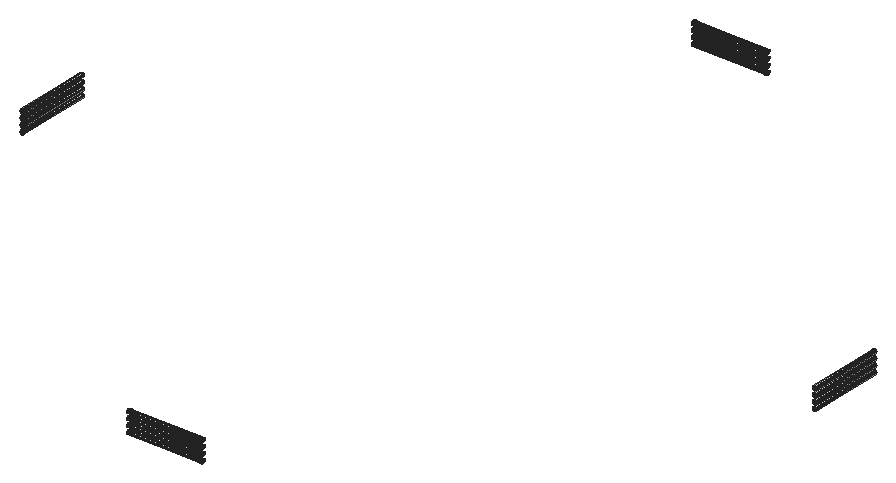
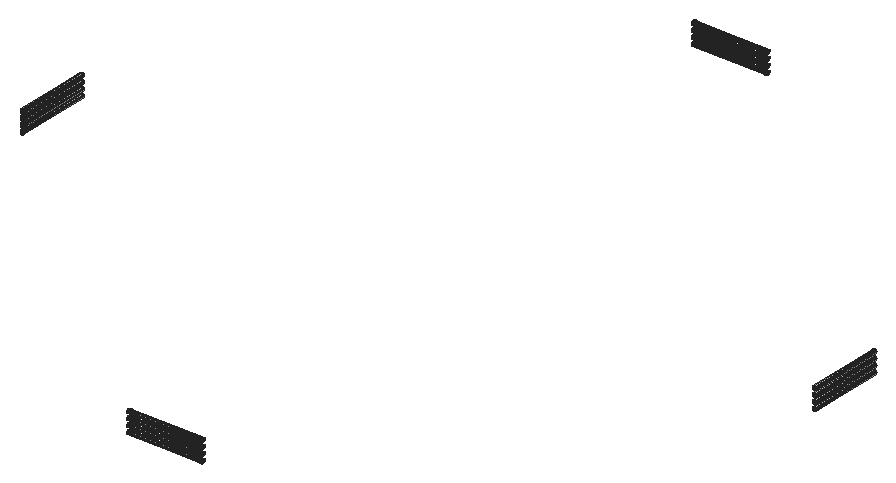
# SketchUp Ruby script. Lengths in inches.
U = 1.inch
M = Sketchup.active_model
def pt(a) = Geom::Point3d.new(a.map { |v| v * U })
def face(e, loops, mat)
  f = e.add_face(loops[0].map { |a| pt(a) })
  loops[1..].each { |l| e.add_face(l.map { |a| pt(a) }).erase! }
  f.material = f.back_material = mat if mat
  f
end
# faces: each face lists its corners as indices into pts; further lists are holes
def faces(e, pts, list, mat = nil) = list.each { |f| face(e, (f[0].is_a?(Array) ? f : [f]).map { |l| l.map { |i| pts[i] } }, mat) }
# xy, xz, yz: faces in a plane at the given z, y or x. An outline is a flat list of corners, or four numbers for a rectangle; further outlines are holes
def ring(l) = l.size == 4 ? [[l[0], l[1]], [l[2], l[1]], [l[2], l[3]], [l[0], l[3]]] : l.each_slice(2).to_a
def flat(e, list, mat, &to3) = list.each { |f| face(e, (f[0].is_a?(Array) ? f : [f]).map { |l| ring(l).map { |u, v| to3.(u, v) } }, mat) }
def xy(e, z, list, mat = nil) = flat(e, list, mat) { |x, y| [x, y, z] }
def xz(e, y, list, mat = nil) = flat(e, list, mat) { |x, z| [x, y, z] }
def yz(e, x, list, mat = nil) = flat(e, list, mat) { |y, z| [x, y, z] }
def lines(e, pts, list) = list.each { |a, b| e.add_line(pt(pts[a]), pt(pts[b])) }
# prism: a flat outline (further loops are holes) pulled along v
def prism(e, loops, v, mat = nil)
  f = face(e, loops, mat); d = Geom::Vector3d.new(v.map { |x| x * U })
  f.pushpull(f.normal.samedirection?(d) ? d.length : -d.length)
end
def box(e, o, s, mat = nil) = prism(e, [[o, [o[0] + s[0], o[1], o[2]], [o[0] + s[0], o[1] + s[1], o[2]], [o[0], o[1] + s[1], o[2]]]], [0, 0, s[2]], mat)
def at(x, y, z, deg = 0) = Geom::Transformation.translation(pt([x, y, z])) * Geom::Transformation.rotation(ORIGIN, Z_AXIS, deg.degrees)
def axes(o, x, y, z) = Geom::Transformation.new([*x, 0, *y, 0, *z, 0, *pt(o).to_a, 1])
def part(name) = M.definitions.add(name)
# library, detail: a bought-in or finely detailed component or shape, given as its bounding box
def library(name, o, s) = part(name).tap { |d| box(d.entities, o, s) }
def detail(e, o, s) = box(e.add_group.entities, o, s)
def put(e, d, t, mat = nil) = e.add_instance(d, t).tap { |i| i.material = mat if mat }
def group(e, t, mat = nil) = e.add_group.tap { |g| g.transformation = t; g.material = mat if mat }.entities
root = M.entities
p = [[922.01,48.34,1269.02],[922.01,47.38,1269.14],[778.64,47.38,1269.14],[778.64,48.34,1269.02],[922.01,49.29,1269.14],[778.64,49.29,1269.14],
  [83.53,662.8,1269.02],[82.57,662.8,1269.14],[82.57,806.17,1269.14],[83.53,806.17,1269.02],[84.48,662.8,1269.14],[84.48,806.17,1269.14],
  [1535.52,886.83,1269.14],[1536.47,886.83,1269.02],[1536.47,743.45,1269.02],[1535.52,743.45,1269.14],[1537.43,886.83,1269.14],[1537.43,743.45,1269.14],
  [697.99,1500.33,1269.14],[697.99,1501.28,1269.02],[841.36,1501.28,1269.02],[841.36,1500.33,1269.14],[697.99,1502.24,1269.14],[841.36,1502.24,1269.14],
  [922.01,46.5,1269.51],[778.64,46.5,1269.51],[922.01,50.18,1269.51],[778.64,50.18,1269.51],[81.68,662.8,1269.51],[81.68,806.17,1269.51],
  [85.37,662.8,1269.51],[85.37,806.17,1269.51],[1534.63,886.83,1269.51],[1534.63,743.45,1269.51],[1538.32,886.83,1269.51],[1538.32,743.45,1269.51],
  [697.99,1499.44,1269.51],[841.36,1499.44,1269.51],[697.99,1503.13,1269.51],[841.36,1503.13,1269.51],[922.01,45.73,1270.1],[778.64,45.73,1270.1],
  [922.01,50.95,1270.1],[778.64,50.95,1270.1],[80.92,662.8,1270.1],[80.92,806.17,1270.1],[86.13,662.8,1270.1],[86.13,806.17,1270.1],
  [1533.87,886.83,1270.1],[1533.87,743.45,1270.1],[1539.08,886.83,1270.1],[1539.08,743.45,1270.1],[697.99,1498.68,1270.1],[841.36,1498.68,1270.1],
  [697.99,1503.89,1270.1],[841.36,1503.89,1270.1],[922.01,45.15,1270.86],[778.64,45.15,1270.86],[922.01,51.53,1270.86],[778.64,51.53,1270.86],
  [80.33,662.8,1270.86],[80.33,806.17,1270.86],[86.72,662.8,1270.86],[86.72,806.17,1270.86],[1533.28,886.83,1270.86],[1533.28,743.45,1270.86],
  [1539.67,886.83,1270.86],[1539.67,743.45,1270.86],[697.99,1498.09,1270.86],[841.36,1498.09,1270.86],[697.99,1504.48,1270.86],[841.36,1504.48,1270.86],
  [922.01,44.78,1271.75],[778.64,44.78,1271.75],[922.01,51.9,1271.75],[778.64,51.9,1271.75],[79.97,662.8,1271.75],[79.97,806.17,1271.75],
  [87.09,662.8,1271.75],[87.09,806.17,1271.75],[1532.91,886.83,1271.75],[1532.91,743.45,1271.75],[1540.03,886.83,1271.75],[1540.03,743.45,1271.75],
  [697.99,1497.72,1271.75],[841.36,1497.72,1271.75],[697.99,1504.85,1271.75],[841.36,1504.85,1271.75],[922.01,44.65,1272.7],[778.64,44.65,1272.7],
  [922.01,52.03,1272.7],[778.64,52.03,1272.7],[79.84,662.8,1272.7],[79.84,806.17,1272.7],[87.21,662.8,1272.7],[87.21,806.17,1272.7],
  [1532.79,886.83,1272.7],[1532.79,743.45,1272.7],[1540.16,886.83,1272.7],[1540.16,743.45,1272.7],[697.99,1497.6,1272.7],[841.36,1497.6,1272.7],
  [697.99,1504.97,1272.7],[841.36,1504.97,1272.7],[922.01,44.78,1273.66],[778.64,44.78,1273.66],[922.01,51.9,1273.66],[778.64,51.9,1273.66],
  [79.97,662.8,1273.66],[79.97,806.17,1273.66],[87.09,662.8,1273.66],[87.09,806.17,1273.66],[1532.91,886.83,1273.66],[1532.91,743.45,1273.66],
  [1540.03,886.83,1273.66],[1540.03,743.45,1273.66],[697.99,1497.72,1273.66],[841.36,1497.72,1273.66],[697.99,1504.85,1273.66],[841.36,1504.85,1273.66],
  [922.01,45.15,1274.55],[778.64,45.15,1274.55],[922.01,51.53,1274.55],[778.64,51.53,1274.55],[80.33,662.8,1274.55],[80.33,806.17,1274.55],
  [86.72,662.8,1274.55],[86.72,806.17,1274.55],[1533.28,886.83,1274.55],[1533.28,743.45,1274.55],[1539.67,886.83,1274.55],[1539.67,743.45,1274.55],
  [697.99,1498.09,1274.55],[841.36,1498.09,1274.55],[697.99,1504.48,1274.55],[841.36,1504.48,1274.55],[922.01,45.73,1275.3125],[778.64,45.73,1275.3125],
  [922.01,50.95,1275.3125],[778.64,50.95,1275.3125],[80.92,662.8,1275.3125],[80.92,806.17,1275.3125],[86.13,662.8,1275.3125],[86.13,806.17,1275.3125],
  [1533.87,886.83,1275.3125],[1533.87,743.45,1275.3125],[1539.08,886.83,1275.3125],[1539.08,743.45,1275.3125],[697.99,1498.68,1275.3125],[841.36,1498.68,1275.3125],
  [697.99,1503.89,1275.3125],[841.36,1503.89,1275.3125],[922.01,46.5,1275.9],[778.64,46.5,1275.9],[922.01,50.18,1275.9],[778.64,50.18,1275.9],
  [81.68,662.8,1275.9],[81.68,806.17,1275.9],[85.37,662.8,1275.9],[85.37,806.17,1275.9],[1534.63,886.83,1275.9],[1534.63,743.45,1275.9],
  [1538.32,886.83,1275.9],[1538.32,743.45,1275.9],[697.99,1499.44,1275.9],[841.36,1499.44,1275.9],[697.99,1503.13,1275.9],[841.36,1503.13,1275.9],
  [922.01,47.38,1276.27],[778.64,47.38,1276.27],[922.01,49.29,1276.27],[778.64,49.29,1276.27],[82.57,662.8,1276.27],[82.57,806.17,1276.27],
  [84.48,662.8,1276.27],[84.48,806.17,1276.27],[1535.52,886.83,1276.27],[1535.52,743.45,1276.27],[1537.43,886.83,1276.27],[1537.43,743.45,1276.27],
  [697.99,1500.33,1276.27],[841.36,1500.33,1276.27],[697.99,1502.24,1276.27],[841.36,1502.24,1276.27],[922.01,48.34,1276.39],[778.64,48.34,1276.39],
  [83.53,662.8,1276.39],[83.53,806.17,1276.39],[1536.47,886.83,1276.39],[1536.47,743.45,1276.39],[697.99,1501.28,1276.39],[841.36,1501.28,1276.39],
  [922.01,48.34,1281.02],[922.01,47.38,1281.14],[778.64,47.38,1281.14],[778.64,48.34,1281.02],[922.01,49.29,1281.14],[778.64,49.29,1281.14],
  [83.53,662.8,1281.02],[82.57,662.8,1281.14],[82.57,806.17,1281.14],[83.53,806.17,1281.02],[84.48,662.8,1281.14],[84.48,806.17,1281.14],
  [1535.52,886.83,1281.14],[1536.47,886.83,1281.02],[1536.47,743.45,1281.02],[1535.52,743.45,1281.14],[1537.43,886.83,1281.14],[1537.43,743.45,1281.14],
  [697.99,1500.33,1281.14],[697.99,1501.28,1281.02],[841.36,1501.28,1281.02],[841.36,1500.33,1281.14],[697.99,1502.24,1281.14],[841.36,1502.24,1281.14],
  [922.01,46.5,1281.51],[778.64,46.5,1281.51],[922.01,50.18,1281.51],[778.64,50.18,1281.51],[81.68,662.8,1281.51],[81.68,806.17,1281.51],
  [85.37,662.8,1281.51],[85.37,806.17,1281.51],[1534.63,886.83,1281.51],[1534.63,743.45,1281.51],[1538.32,886.83,1281.51],[1538.32,743.45,1281.51],
  [697.99,1499.44,1281.51],[841.36,1499.44,1281.51],[697.99,1503.13,1281.51],[841.36,1503.13,1281.51],[922.01,45.73,1282.1],[778.64,45.73,1282.1],
  [922.01,50.95,1282.1],[778.64,50.95,1282.1],[80.92,662.8,1282.1],[80.92,806.17,1282.1],[86.13,662.8,1282.1],[86.13,806.17,1282.1],
  [1533.87,886.83,1282.1],[1533.87,743.45,1282.1],[1539.08,886.83,1282.1],[1539.08,743.45,1282.1],[697.99,1498.68,1282.1],[841.36,1498.68,1282.1],
  [697.99,1503.89,1282.1],[841.36,1503.89,1282.1],[922.01,45.15,1282.86],[778.64,45.15,1282.86],[922.01,51.53,1282.86],[778.64,51.53,1282.86],
  [80.33,662.8,1282.86],[80.33,806.17,1282.86],[86.72,662.8,1282.86],[86.72,806.17,1282.86],[1533.28,886.83,1282.86],[1533.28,743.45,1282.86],
  [1539.67,886.83,1282.86],[1539.67,743.45,1282.86],[697.99,1498.09,1282.86],[841.36,1498.09,1282.86],[697.99,1504.48,1282.86],[841.36,1504.48,1282.86],
  [922.01,44.78,1283.75],[778.64,44.78,1283.75],[922.01,51.9,1283.75],[778.64,51.9,1283.75],[79.97,662.8,1283.75],[79.97,806.17,1283.75],
  [87.09,662.8,1283.75],[87.09,806.17,1283.75],[1532.91,886.83,1283.75],[1532.91,743.45,1283.75],[1540.03,886.83,1283.75],[1540.03,743.45,1283.75],
  [697.99,1497.72,1283.75],[841.36,1497.72,1283.75],[697.99,1504.85,1283.75],[841.36,1504.85,1283.75],[922.01,44.65,1284.7],[778.64,44.65,1284.7],
  [922.01,52.03,1284.7],[778.64,52.03,1284.7],[79.84,662.8,1284.7],[79.84,806.17,1284.7],[87.21,662.8,1284.7],[87.21,806.17,1284.7],
  [1532.79,886.83,1284.7],[1532.79,743.45,1284.7],[1540.16,886.83,1284.7],[1540.16,743.45,1284.7],[697.99,1497.6,1284.7],[841.36,1497.6,1284.7],
  [697.99,1504.97,1284.7],[841.36,1504.97,1284.7],[922.01,44.78,1285.66],[778.64,44.78,1285.66],[922.01,51.9,1285.66],[778.64,51.9,1285.66],
  [79.97,662.8,1285.66],[79.97,806.17,1285.66],[87.09,662.8,1285.66],[87.09,806.17,1285.66],[1532.91,886.83,1285.66],[1532.91,743.45,1285.66],
  [1540.03,886.83,1285.66],[1540.03,743.45,1285.66],[697.99,1497.72,1285.66],[841.36,1497.72,1285.66],[697.99,1504.85,1285.66],[841.36,1504.85,1285.66],
  [922.01,45.15,1286.55],[778.64,45.15,1286.55],[922.01,51.53,1286.55],[778.64,51.53,1286.55],[80.33,662.8,1286.55],[80.33,806.17,1286.55],
  [86.72,662.8,1286.55],[86.72,806.17,1286.55],[1533.28,886.83,1286.55],[1533.28,743.45,1286.55],[1539.67,886.83,1286.55],[1539.67,743.45,1286.55],
  [697.99,1498.09,1286.55],[841.36,1498.09,1286.55],[697.99,1504.48,1286.55],[841.36,1504.48,1286.55],[922.01,45.73,1287.3125],[778.64,45.73,1287.3125],
  [922.01,50.95,1287.3125],[778.64,50.95,1287.3125],[80.92,662.8,1287.3125],[80.92,806.17,1287.3125],[86.13,662.8,1287.3125],[86.13,806.17,1287.3125],
  [1533.87,886.83,1287.3125],[1533.87,743.45,1287.3125],[1539.08,886.83,1287.3125],[1539.08,743.45,1287.3125],[697.99,1498.68,1287.3125],[841.36,1498.68,1287.3125],
  [697.99,1503.89,1287.3125],[841.36,1503.89,1287.3125],[922.01,46.5,1287.9],[778.64,46.5,1287.9],[922.01,50.18,1287.9],[778.64,50.18,1287.9],
  [81.68,662.8,1287.9],[81.68,806.17,1287.9],[85.37,662.8,1287.9],[85.37,806.17,1287.9],[1534.63,886.83,1287.9],[1534.63,743.45,1287.9],
  [1538.32,886.83,1287.9],[1538.32,743.45,1287.9],[697.99,1499.44,1287.9],[841.36,1499.44,1287.9],[697.99,1503.13,1287.9],[841.36,1503.13,1287.9],
  [922.01,47.38,1288.27],[778.64,47.38,1288.27],[922.01,49.29,1288.27],[778.64,49.29,1288.27],[82.57,662.8,1288.27],[82.57,806.17,1288.27],
  [84.48,662.8,1288.27],[84.48,806.17,1288.27],[1535.52,886.83,1288.27],[1535.52,743.45,1288.27],[1537.43,886.83,1288.27],[1537.43,743.45,1288.27],
  [697.99,1500.33,1288.27],[841.36,1500.33,1288.27],[697.99,1502.24,1288.27],[841.36,1502.24,1288.27],[922.01,48.34,1288.39],[778.64,48.34,1288.39],
  [83.53,662.8,1288.39],[83.53,806.17,1288.39],[1536.47,886.83,1288.39],[1536.47,743.45,1288.39],[697.99,1501.28,1288.39],[841.36,1501.28,1288.39],
  [922.01,48.34,1293.02],[922.01,47.38,1293.14],[778.64,47.38,1293.14],[778.64,48.34,1293.02],[922.01,49.29,1293.14],[778.64,49.29,1293.14],
  [83.53,662.8,1293.02],[82.57,662.8,1293.14],[82.57,806.17,1293.14],[83.53,806.17,1293.02],[84.48,662.8,1293.14],[84.48,806.17,1293.14],
  [1535.52,886.83,1293.14],[1536.47,886.83,1293.02],[1536.47,743.45,1293.02],[1535.52,743.45,1293.14],[1537.43,886.83,1293.14],[1537.43,743.45,1293.14],
  [697.99,1500.33,1293.14],[697.99,1501.28,1293.02],[841.36,1501.28,1293.02],[841.36,1500.33,1293.14],[697.99,1502.24,1293.14],[841.36,1502.24,1293.14],
  [922.01,46.5,1293.51],[778.64,46.5,1293.51],[922.01,50.18,1293.51],[778.64,50.18,1293.51],[81.68,662.8,1293.51],[81.68,806.17,1293.51],
  [85.37,662.8,1293.51],[85.37,806.17,1293.51],[1534.63,886.83,1293.51],[1534.63,743.45,1293.51],[1538.32,886.83,1293.51],[1538.32,743.45,1293.51],
  [697.99,1499.44,1293.51],[841.36,1499.44,1293.51],[697.99,1503.13,1293.51],[841.36,1503.13,1293.51],[922.01,45.73,1294.1],[778.64,45.73,1294.1],
  [922.01,50.95,1294.1],[778.64,50.95,1294.1],[80.92,662.8,1294.1],[80.92,806.17,1294.1],[86.13,662.8,1294.1],[86.13,806.17,1294.1],
  [1533.87,886.83,1294.1],[1533.87,743.45,1294.1],[1539.08,886.83,1294.1],[1539.08,743.45,1294.1],[697.99,1498.68,1294.1],[841.36,1498.68,1294.1],
  [697.99,1503.89,1294.1],[841.36,1503.89,1294.1],[922.01,45.15,1294.86],[778.64,45.15,1294.86],[922.01,51.53,1294.86],[778.64,51.53,1294.86],
  [80.33,662.8,1294.86],[80.33,806.17,1294.86],[86.72,662.8,1294.86],[86.72,806.17,1294.86],[1533.28,886.83,1294.86],[1533.28,743.45,1294.86],
  [1539.67,886.83,1294.86],[1539.67,743.45,1294.86],[697.99,1498.09,1294.86],[841.36,1498.09,1294.86],[697.99,1504.48,1294.86],[841.36,1504.48,1294.86],
  [922.01,44.78,1295.75],[778.64,44.78,1295.75],[922.01,51.9,1295.75],[778.64,51.9,1295.75],[79.97,662.8,1295.75],[79.97,806.17,1295.75],
  [87.09,662.8,1295.75],[87.09,806.17,1295.75],[1532.91,886.83,1295.75],[1532.91,743.45,1295.75],[1540.03,886.83,1295.75],[1540.03,743.45,1295.75],
  [697.99,1497.72,1295.75],[841.36,1497.72,1295.75],[697.99,1504.85,1295.75],[841.36,1504.85,1295.75],[922.01,44.65,1296.7],[778.64,44.65,1296.7],
  [922.01,52.03,1296.7],[778.64,52.03,1296.7],[79.84,662.8,1296.7],[79.84,806.17,1296.7],[87.21,662.8,1296.7],[87.21,806.17,1296.7],
  [1532.79,886.83,1296.7],[1532.79,743.45,1296.7],[1540.16,886.83,1296.7],[1540.16,743.45,1296.7],[697.99,1497.6,1296.7],[841.36,1497.6,1296.7],
  [697.99,1504.97,1296.7],[841.36,1504.97,1296.7],[922.01,44.78,1297.66],[778.64,44.78,1297.66],[922.01,51.9,1297.66],[778.64,51.9,1297.66],
  [79.97,662.8,1297.66],[79.97,806.17,1297.66],[87.09,662.8,1297.66],[87.09,806.17,1297.66],[1532.91,886.83,1297.66],[1532.91,743.45,1297.66],
  [1540.03,886.83,1297.66],[1540.03,743.45,1297.66],[697.99,1497.72,1297.66],[841.36,1497.72,1297.66],[697.99,1504.85,1297.66],[841.36,1504.85,1297.66],
  [922.01,45.15,1298.55],[778.64,45.15,1298.55],[922.01,51.53,1298.55],[778.64,51.53,1298.55],[80.33,662.8,1298.55],[80.33,806.17,1298.55],
  [86.72,662.8,1298.55],[86.72,806.17,1298.55],[1533.28,886.83,1298.55],[1533.28,743.45,1298.55],[1539.67,886.83,1298.55],[1539.67,743.45,1298.55],
  [697.99,1498.09,1298.55],[841.36,1498.09,1298.55],[697.99,1504.48,1298.55],[841.36,1504.48,1298.55],[922.01,45.73,1299.3125],[778.64,45.73,1299.3125],
  [922.01,50.95,1299.3125],[778.64,50.95,1299.3125],[80.92,662.8,1299.3125],[80.92,806.17,1299.3125],[86.13,662.8,1299.3125],[86.13,806.17,1299.3125],
  [1533.87,886.83,1299.3125],[1533.87,743.45,1299.3125],[1539.08,886.83,1299.3125],[1539.08,743.45,1299.3125],[697.99,1498.68,1299.3125],[841.36,1498.68,1299.3125],
  [697.99,1503.89,1299.3125],[841.36,1503.89,1299.3125],[922.01,46.5,1299.9],[778.64,46.5,1299.9],[922.01,50.18,1299.9],[778.64,50.18,1299.9],
  [81.68,662.8,1299.9],[81.68,806.17,1299.9],[85.37,662.8,1299.9],[85.37,806.17,1299.9],[1534.63,886.83,1299.9],[1534.63,743.45,1299.9],
  [1538.32,886.83,1299.9],[1538.32,743.45,1299.9],[697.99,1499.44,1299.9],[841.36,1499.44,1299.9],[697.99,1503.13,1299.9],[841.36,1503.13,1299.9],
  [922.01,47.38,1300.27],[778.64,47.38,1300.27],[922.01,49.29,1300.27],[778.64,49.29,1300.27],[82.57,662.8,1300.27],[82.57,806.17,1300.27],
  [84.48,662.8,1300.27],[84.48,806.17,1300.27],[1535.52,886.83,1300.27],[1535.52,743.45,1300.27],[1537.43,886.83,1300.27],[1537.43,743.45,1300.27],
  [697.99,1500.33,1300.27],[841.36,1500.33,1300.27],[697.99,1502.24,1300.27],[841.36,1502.24,1300.27],[922.01,48.34,1300.39],[778.64,48.34,1300.39],
  [83.53,662.8,1300.39],[83.53,806.17,1300.39],[1536.47,886.83,1300.39],[1536.47,743.45,1300.39],[697.99,1501.28,1300.39],[841.36,1501.28,1300.39],
  [922.01,48.34,1305.02],[922.01,47.38,1305.14],[778.64,47.38,1305.14],[778.64,48.34,1305.02],[922.01,49.29,1305.14],[778.64,49.29,1305.14],
  [83.53,662.8,1305.02],[82.57,662.8,1305.14],[82.57,806.17,1305.14],[83.53,806.17,1305.02],[84.48,662.8,1305.14],[84.48,806.17,1305.14],
  [1535.52,886.83,1305.14],[1536.47,886.83,1305.02],[1536.47,743.45,1305.02],[1535.52,743.45,1305.14],[1537.43,886.83,1305.14],[1537.43,743.45,1305.14],
  [697.99,1500.33,1305.14],[697.99,1501.28,1305.02],[841.36,1501.28,1305.02],[841.36,1500.33,1305.14],[697.99,1502.24,1305.14],[841.36,1502.24,1305.14],
  [922.01,46.5,1305.51],[778.64,46.5,1305.51],[922.01,50.18,1305.51],[778.64,50.18,1305.51],[81.68,662.8,1305.51],[81.68,806.17,1305.51],
  [85.37,662.8,1305.51],[85.37,806.17,1305.51],[1534.63,886.83,1305.51],[1534.63,743.45,1305.51],[1538.32,886.83,1305.51],[1538.32,743.45,1305.51],
  [697.99,1499.44,1305.51],[841.36,1499.44,1305.51],[697.99,1503.13,1305.51],[841.36,1503.13,1305.51],[922.01,45.73,1306.1],[778.64,45.73,1306.1],
  [922.01,50.95,1306.1],[778.64,50.95,1306.1],[80.92,662.8,1306.1],[80.92,806.17,1306.1],[86.13,662.8,1306.1],[86.13,806.17,1306.1],
  [1533.87,886.83,1306.1],[1533.87,743.45,1306.1],[1539.08,886.83,1306.1],[1539.08,743.45,1306.1],[697.99,1498.68,1306.1],[841.36,1498.68,1306.1],
  [697.99,1503.89,1306.1],[841.36,1503.89,1306.1],[922.01,45.15,1306.86],[778.64,45.15,1306.86],[922.01,51.53,1306.86],[778.64,51.53,1306.86],
  [80.33,662.8,1306.86],[80.33,806.17,1306.86],[86.72,662.8,1306.86],[86.72,806.17,1306.86],[1533.28,886.83,1306.86],[1533.28,743.45,1306.86],
  [1539.67,886.83,1306.86],[1539.67,743.45,1306.86],[697.99,1498.09,1306.86],[841.36,1498.09,1306.86],[697.99,1504.48,1306.86],[841.36,1504.48,1306.86],
  [922.01,44.78,1307.75],[778.64,44.78,1307.75],[922.01,51.9,1307.75],[778.64,51.9,1307.75],[79.97,662.8,1307.75],[79.97,806.17,1307.75],
  [87.09,662.8,1307.75],[87.09,806.17,1307.75],[1532.91,886.83,1307.75],[1532.91,743.45,1307.75],[1540.03,886.83,1307.75],[1540.03,743.45,1307.75],
  [697.99,1497.72,1307.75],[841.36,1497.72,1307.75],[697.99,1504.85,1307.75],[841.36,1504.85,1307.75],[922.01,44.65,1308.7],[778.64,44.65,1308.7],
  [922.01,52.03,1308.7],[778.64,52.03,1308.7],[79.84,662.8,1308.7],[79.84,806.17,1308.7],[87.21,662.8,1308.7],[87.21,806.17,1308.7],
  [1532.79,886.83,1308.7],[1532.79,743.45,1308.7],[1540.16,886.83,1308.7],[1540.16,743.45,1308.7],[697.99,1497.6,1308.7],[841.36,1497.6,1308.7],
  [697.99,1504.97,1308.7],[841.36,1504.97,1308.7],[922.01,44.78,1309.66],[778.64,44.78,1309.66],[922.01,51.9,1309.66],[778.64,51.9,1309.66],
  [79.97,662.8,1309.66],[79.97,806.17,1309.66],[87.09,662.8,1309.66],[87.09,806.17,1309.66],[1532.91,886.83,1309.66],[1532.91,743.45,1309.66],
  [1540.03,886.83,1309.66],[1540.03,743.45,1309.66],[697.99,1497.72,1309.66],[841.36,1497.72,1309.66],[697.99,1504.85,1309.66],[841.36,1504.85,1309.66],
  [922.01,45.15,1310.55],[778.64,45.15,1310.55],[922.01,51.53,1310.55],[778.64,51.53,1310.55],[80.33,662.8,1310.55],[80.33,806.17,1310.55],
  [86.72,662.8,1310.55],[86.72,806.17,1310.55],[1533.28,886.83,1310.55],[1533.28,743.45,1310.55],[1539.67,886.83,1310.55],[1539.67,743.45,1310.55],
  [697.99,1498.09,1310.55],[841.36,1498.09,1310.55],[697.99,1504.48,1310.55],[841.36,1504.48,1310.55],[922.01,45.73,1311.3125],[778.64,45.73,1311.3125],
  [922.01,50.95,1311.3125],[778.64,50.95,1311.3125],[80.92,662.8,1311.3125],[80.92,806.17,1311.3125],[86.13,662.8,1311.3125],[86.13,806.17,1311.3125],
  [1533.87,886.83,1311.3125],[1533.87,743.45,1311.3125],[1539.08,886.83,1311.3125],[1539.08,743.45,1311.3125],[697.99,1498.68,1311.3125],[841.36,1498.68,1311.3125],
  [697.99,1503.89,1311.3125],[841.36,1503.89,1311.3125],[922.01,46.5,1311.9],[778.64,46.5,1311.9],[922.01,50.18,1311.9],[778.64,50.18,1311.9],
  [81.68,662.8,1311.9],[81.68,806.17,1311.9],[85.37,662.8,1311.9],[85.37,806.17,1311.9],[1534.63,886.83,1311.9],[1534.63,743.45,1311.9],
  [1538.32,886.83,1311.9],[1538.32,743.45,1311.9],[697.99,1499.44,1311.9],[841.36,1499.44,1311.9],[697.99,1503.13,1311.9],[841.36,1503.13,1311.9],
  [922.01,47.38,1312.27],[778.64,47.38,1312.27],[922.01,49.29,1312.27],[778.64,49.29,1312.27],[82.57,662.8,1312.27],[82.57,806.17,1312.27],
  [84.48,662.8,1312.27],[84.48,806.17,1312.27],[1535.52,886.83,1312.27],[1535.52,743.45,1312.27],[1537.43,886.83,1312.27],[1537.43,743.45,1312.27],
  [697.99,1500.33,1312.27],[841.36,1500.33,1312.27],[697.99,1502.24,1312.27],[841.36,1502.24,1312.27],[922.01,48.34,1312.39],[778.64,48.34,1312.39],
  [83.53,662.8,1312.39],[83.53,806.17,1312.39],[1536.47,886.83,1312.39],[1536.47,743.45,1312.39],[697.99,1501.28,1312.39],[841.36,1501.28,1312.39]]
faces(root,p,[[0,1,2,3],[4,0,3,5],[6,7,8,9],[10,6,9,11],[12,13,14,15],[13,16,17,14],[18,19,20,21],[19,22,23,20],
  [1,24,25,2],[26,4,5,27],[7,28,29,8],[30,10,11,31],[32,12,15,33],[16,34,35,17],[36,18,21,37],[22,38,39,23],
  [24,40,41,25],[42,26,27,43],[28,44,45,29],[46,30,31,47],[48,32,33,49],[34,50,51,35],[52,36,37,53],[38,54,55,39],
  [40,56,57,41],[58,42,43,59],[44,60,61,45],[62,46,47,63],[64,48,49,65],[50,66,67,51],[68,52,53,69],[54,70,71,55],
  [56,72,73,57],[74,58,59,75],[60,76,77,61],[78,62,63,79],[80,64,65,81],[66,82,83,67],[84,68,69,85],[70,86,87,71],
  [72,88,89,73],[90,74,75,91],[76,92,93,77],[94,78,79,95],[96,80,81,97],[82,98,99,83],[100,84,85,101],[86,102,103,87],
  [88,104,105,89],[106,90,91,107],[92,108,109,93],[110,94,95,111],[112,96,97,113],[98,114,115,99],[116,100,101,117],[102,118,119,103],
  [104,120,121,105],[122,106,107,123],[108,124,125,109],[126,110,111,127],[128,112,113,129],[114,130,131,115],[132,116,117,133],[118,134,135,119],
  [120,136,137,121],[138,122,123,139],[124,140,141,125],[142,126,127,143],[144,128,129,145],[130,146,147,131],[148,132,133,149],[134,150,151,135],
  [136,152,153,137],[154,138,139,155],[140,156,157,141],[158,142,143,159],[160,144,145,161],[146,162,163,147],[164,148,149,165],[150,166,167,151],
  [152,168,169,153],[170,154,155,171],[156,172,173,157],[174,158,159,175],[176,160,161,177],[162,178,179,163],[180,164,165,181],[166,182,183,167],
  [168,184,185,169],[184,170,171,185],[172,186,187,173],[186,174,175,187],[188,176,177,189],[178,188,189,179],[190,180,181,191],[182,190,191,183],
  [192,193,194,195],[196,192,195,197],[198,199,200,201],[202,198,201,203],[204,205,206,207],[205,208,209,206],[210,211,212,213],[211,214,215,212],
  [193,216,217,194],[218,196,197,219],[199,220,221,200],[222,202,203,223],[224,204,207,225],[208,226,227,209],[228,210,213,229],[214,230,231,215],
  [216,232,233,217],[234,218,219,235],[220,236,237,221],[238,222,223,239],[240,224,225,241],[226,242,243,227],[244,228,229,245],[230,246,247,231],
  [232,248,249,233],[250,234,235,251],[236,252,253,237],[254,238,239,255],[256,240,241,257],[242,258,259,243],[260,244,245,261],[246,262,263,247],
  [248,264,265,249],[266,250,251,267],[252,268,269,253],[270,254,255,271],[272,256,257,273],[258,274,275,259],[276,260,261,277],[262,278,279,263],
  [264,280,281,265],[282,266,267,283],[268,284,285,269],[286,270,271,287],[288,272,273,289],[274,290,291,275],[292,276,277,293],[278,294,295,279],
  [280,296,297,281],[298,282,283,299],[284,300,301,285],[302,286,287,303],[304,288,289,305],[290,306,307,291],[308,292,293,309],[294,310,311,295],
  [296,312,313,297],[314,298,299,315],[300,316,317,301],[318,302,303,319],[320,304,305,321],[306,322,323,307],[324,308,309,325],[310,326,327,311],
  [312,328,329,313],[330,314,315,331],[316,332,333,317],[334,318,319,335],[336,320,321,337],[322,338,339,323],[340,324,325,341],[326,342,343,327],
  [328,344,345,329],[346,330,331,347],[332,348,349,333],[350,334,335,351],[352,336,337,353],[338,354,355,339],[356,340,341,357],[342,358,359,343],
  [344,360,361,345],[362,346,347,363],[348,364,365,349],[366,350,351,367],[368,352,353,369],[354,370,371,355],[372,356,357,373],[358,374,375,359],
  [360,376,377,361],[376,362,363,377],[364,378,379,365],[378,366,367,379],[380,368,369,381],[370,380,381,371],[382,372,373,383],[374,382,383,375],
  [384,385,386,387],[388,384,387,389],[390,391,392,393],[394,390,393,395],[396,397,398,399],[397,400,401,398],[402,403,404,405],[403,406,407,404],
  [385,408,409,386],[410,388,389,411],[391,412,413,392],[414,394,395,415],[416,396,399,417],[400,418,419,401],[420,402,405,421],[406,422,423,407],
  [408,424,425,409],[426,410,411,427],[412,428,429,413],[430,414,415,431],[432,416,417,433],[418,434,435,419],[436,420,421,437],[422,438,439,423],
  [424,440,441,425],[442,426,427,443],[428,444,445,429],[446,430,431,447],[448,432,433,449],[434,450,451,435],[452,436,437,453],[438,454,455,439],
  [440,456,457,441],[458,442,443,459],[444,460,461,445],[462,446,447,463],[464,448,449,465],[450,466,467,451],[468,452,453,469],[454,470,471,455],
  [456,472,473,457],[474,458,459,475],[460,476,477,461],[478,462,463,479],[480,464,465,481],[466,482,483,467],[484,468,469,485],[470,486,487,471],
  [472,488,489,473],[490,474,475,491],[476,492,493,477],[494,478,479,495],[496,480,481,497],[482,498,499,483],[500,484,485,501],[486,502,503,487],
  [488,504,505,489],[506,490,491,507],[492,508,509,493],[510,494,495,511],[512,496,497,513],[498,514,515,499],[516,500,501,517],[502,518,519,503],
  [504,520,521,505],[522,506,507,523],[508,524,525,509],[526,510,511,527],[528,512,513,529],[514,530,531,515],[532,516,517,533],[518,534,535,519],
  [520,536,537,521],[538,522,523,539],[524,540,541,525],[542,526,527,543],[544,528,529,545],[530,546,547,531],[548,532,533,549],[534,550,551,535],
  [536,552,553,537],[554,538,539,555],[540,556,557,541],[558,542,543,559],[560,544,545,561],[546,562,563,547],[564,548,549,565],[550,566,567,551],
  [552,568,569,553],[568,554,555,569],[556,570,571,557],[570,558,559,571],[572,560,561,573],[562,572,573,563],[574,564,565,575],[566,574,575,567],
  [576,577,578,579],[580,576,579,581],[582,583,584,585],[586,582,585,587],[588,589,590,591],[589,592,593,590],[594,595,596,597],[595,598,599,596],
  [577,600,601,578],[602,580,581,603],[583,604,605,584],[606,586,587,607],[608,588,591,609],[592,610,611,593],[612,594,597,613],[598,614,615,599],
  [600,616,617,601],[618,602,603,619],[604,620,621,605],[622,606,607,623],[624,608,609,625],[610,626,627,611],[628,612,613,629],[614,630,631,615],
  [616,632,633,617],[634,618,619,635],[620,636,637,621],[638,622,623,639],[640,624,625,641],[626,642,643,627],[644,628,629,645],[630,646,647,631],
  [632,648,649,633],[650,634,635,651],[636,652,653,637],[654,638,639,655],[656,640,641,657],[642,658,659,643],[660,644,645,661],[646,662,663,647],
  [648,664,665,649],[666,650,651,667],[652,668,669,653],[670,654,655,671],[672,656,657,673],[658,674,675,659],[676,660,661,677],[662,678,679,663],
  [664,680,681,665],[682,666,667,683],[668,684,685,669],[686,670,671,687],[688,672,673,689],[674,690,691,675],[692,676,677,693],[678,694,695,679],
  [680,696,697,681],[698,682,683,699],[684,700,701,685],[702,686,687,703],[704,688,689,705],[690,706,707,691],[708,692,693,709],[694,710,711,695],
  [696,712,713,697],[714,698,699,715],[700,716,717,701],[718,702,703,719],[720,704,705,721],[706,722,723,707],[724,708,709,725],[710,726,727,711],
  [712,728,729,713],[730,714,715,731],[716,732,733,717],[734,718,719,735],[736,720,721,737],[722,738,739,723],[740,724,725,741],[726,742,743,727],
  [728,744,745,729],[746,730,731,747],[732,748,749,733],[750,734,735,751],[752,736,737,753],[738,754,755,739],[756,740,741,757],[742,758,759,743],
  [744,760,761,745],[760,746,747,761],[748,762,763,749],[762,750,751,763],[764,752,753,765],[754,764,765,755],[766,756,757,767],[758,766,767,759]])
